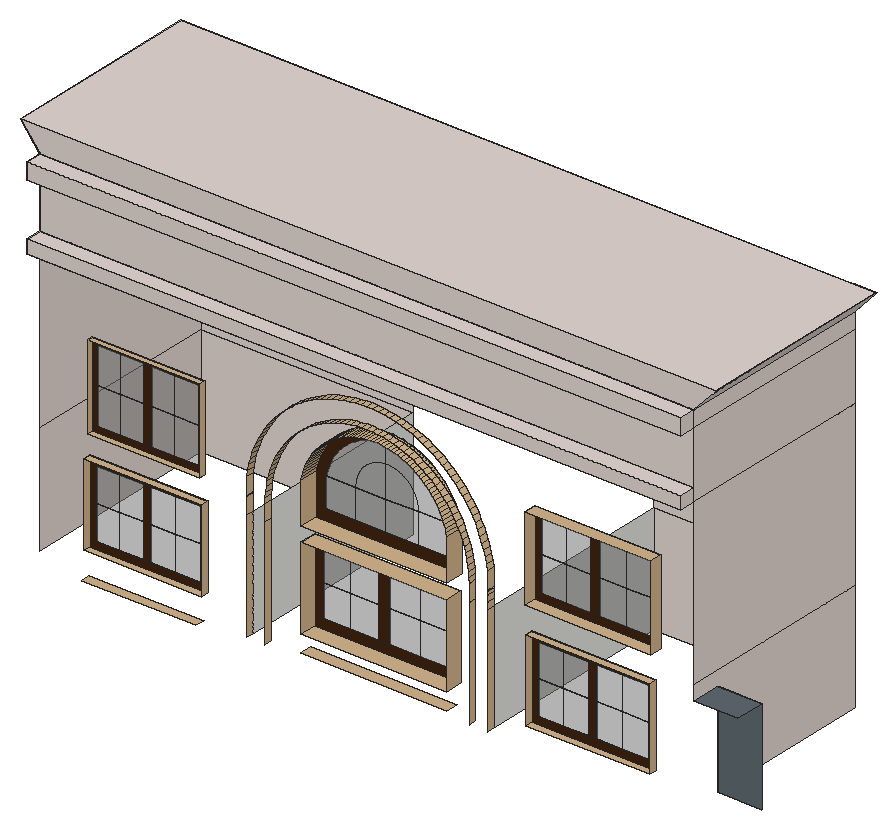
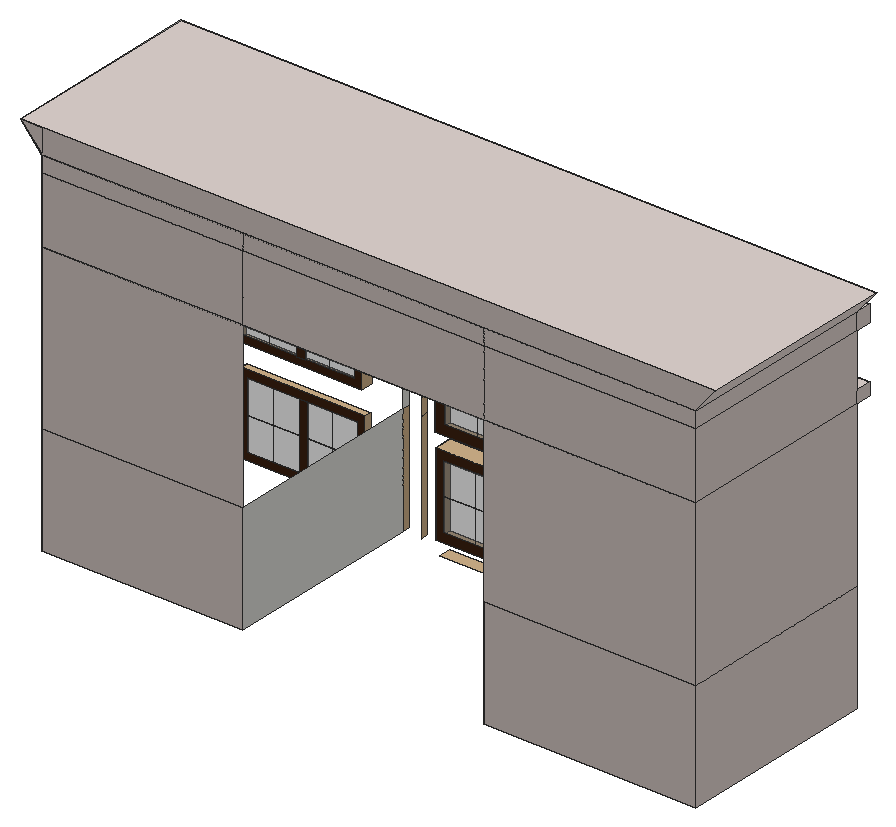
# SketchUp Ruby script. Lengths in inches.
U = 1.inch
M = Sketchup.active_model
def pt(a) = Geom::Point3d.new(a.map { |v| v * U })
def face(e, loops, mat)
  f = e.add_face(loops[0].map { |a| pt(a) })
  loops[1..].each { |l| e.add_face(l.map { |a| pt(a) }).erase! }
  f.material = f.back_material = mat if mat
  f
end
# faces: each face lists its corners as indices into pts; further lists are holes
def faces(e, pts, list, mat = nil) = list.each { |f| face(e, (f[0].is_a?(Array) ? f : [f]).map { |l| l.map { |i| pts[i] } }, mat) }
# xy, xz, yz: faces in a plane at the given z, y or x. An outline is a flat list of corners, or four numbers for a rectangle; further outlines are holes
def ring(l) = l.size == 4 ? [[l[0], l[1]], [l[2], l[1]], [l[2], l[3]], [l[0], l[3]]] : l.each_slice(2).to_a
def flat(e, list, mat, &to3) = list.each { |f| face(e, (f[0].is_a?(Array) ? f : [f]).map { |l| ring(l).map { |u, v| to3.(u, v) } }, mat) }
def xy(e, z, list, mat = nil) = flat(e, list, mat) { |x, y| [x, y, z] }
def xz(e, y, list, mat = nil) = flat(e, list, mat) { |x, z| [x, y, z] }
def yz(e, x, list, mat = nil) = flat(e, list, mat) { |y, z| [x, y, z] }
def lines(e, pts, list) = list.each { |a, b| e.add_line(pt(pts[a]), pt(pts[b])) }
# prism: a flat outline (further loops are holes) pulled along v
def prism(e, loops, v, mat = nil)
  f = face(e, loops, mat); d = Geom::Vector3d.new(v.map { |x| x * U })
  f.pushpull(f.normal.samedirection?(d) ? d.length : -d.length)
end
def box(e, o, s, mat = nil) = prism(e, [[o, [o[0] + s[0], o[1], o[2]], [o[0] + s[0], o[1] + s[1], o[2]], [o[0], o[1] + s[1], o[2]]]], [0, 0, s[2]], mat)
def at(x, y, z, deg = 0) = Geom::Transformation.translation(pt([x, y, z])) * Geom::Transformation.rotation(ORIGIN, Z_AXIS, deg.degrees)
def axes(o, x, y, z) = Geom::Transformation.new([*x, 0, *y, 0, *z, 0, *pt(o).to_a, 1])
def part(name) = M.definitions.add(name)
# library, detail: a bought-in or finely detailed component or shape, given as its bounding box
def library(name, o, s) = part(name).tap { |d| box(d.entities, o, s) }
def detail(e, o, s) = box(e.add_group.entities, o, s)
def put(e, d, t, mat = nil) = e.add_instance(d, t).tap { |i| i.material = mat if mat }
def group(e, t, mat = nil) = e.add_group.tap { |g| g.transformation = t; g.material = mat if mat }.entities
root = M.entities
M.materials.add("[0035_Tan]").color = [210, 180, 140]
M.materials.add("[Concrete Block 8x8 Gray]").color = [226, 214, 209]
M.materials.add("[Formica Speckled Grey]").color = [94, 105, 111]
M.materials.add("[Translucent Glass Gray]").color = [128, 128, 128]
M.materials["[Translucent Glass Gray]"].alpha = 0.5
M.materials.add("[Wood Cherry Original]").color = [66, 37, 18]
M.materials.add("[Wood Cherry Original]1").color = [66, 37, 18]
xy(root,250.26,[[47.15,148.73,134.71,155.98]],"[0035_Tan]")
xy(root,259.4,[[215.4,148.73,327.53,158.04]],"[0035_Tan]")
xy(root,270.29,[[387.81,148.73,483.43,154.29]],"[0035_Tan]")
xy(root,271.61,[[48.61,148.73,139.11,154.35]],"[0035_Tan]")
xy(root,272.4,[[215.4,148.73,327.53,162.23]],"[0035_Tan]")
xy(root,332.73,[[387.81,148.73,483.43,154.29]],"[0035_Tan]")
xy(root,332.73,[[516.88,148.73,550.94,171.42]],"[Formica Speckled Grey]")
xy(root,334.67,[[48.61,148.73,139.11,154.35]],"[0035_Tan]")
xy(root,335.78,[[215.4,148.73,327.53,162.23]],"[0035_Tan]")
xy(root,346.9,[[215.4,148.73,327.53,163.17]],"[0035_Tan]")
xy(root,352.68,[[387.3,148.73,484.24,158.23]],"[0035_Tan]")
xy(root,352.89,[[51.46,148.73,137.53,153.48]],"[0035_Tan]")
xy(root,417.08,[[51.46,148.73,137.53,153.48]],"[0035_Tan]")
xy(root,417.24,[[387.3,148.73,484.24,158.23]],"[0035_Tan]")
xy(root,469.3125,[[15.125,148.73,516.88,302.95]])
xy(root,469.3125,[[15.125,136.17,516.88,148.73]],"[Concrete Block 8x8 Gray]")
xy(root,479.24,[[15.125,136.17,516.88,148.73]],"[Concrete Block 8x8 Gray]")
xy(root,519.9375,[[15.125,136.17,516.88,148.73],[15.125,148.73,516.88,302.95]])
xy(root,532.5625,[[15.125,148.73,516.88,302.95]])
xy(root,532.5625,[[15.125,136.17,516.88,148.73]],"[Concrete Block 8x8 Gray]")
xy(root,551.1875,[[533.63,148.73,533.65,302.95]])
xy(root,551.375,[[0,148.73,533.63,302.95]],"[Concrete Block 8x8 Gray]")
xz(root,136.17,[[15.125,469.3125,516.88,479.24],[15.125,519.9375,516.88,532.5625]],"[Concrete Block 8x8 Gray]")
xz(root,148.73,[[178.17,343.6875,178.15,356.6,177.97,353.85,177.93,348.77],[178.17,343.6875,178.17,356.93,178.15,356.6],[363.16,343.6875,363.18,356.6,363.16,356.93],[363.16,343.6875,363.39,348.77,363.35,353.85,363.18,356.6],[178.15,356.6,178.17,356.93,178.17,370.47,178.125,370.32],
  [363.18,356.6,363.2,370.32,363.16,370.47,363.16,356.93],[15.125,469.3125,516.88,479.24],[15.125,519.9375,516.88,532.5625]])
xz(root,148.73,[[15.125,479.24,516.88,519.9375],[15.125,532.5625,516.88,532.5625,533.65,551.1875,533.63,551.1875,533.63,551.375,0,551.375]],"[Concrete Block 8x8 Gray]")
xz(root,153.48,[[55.61,357.04,73.22,384.98],[73.22,357.04,90.83,384.98],[96.95,357.04,115.16,384.98],[115.16,357.04,133.38,384.98],[55.61,384.98,73.22,412.93],
  [73.22,384.98,90.83,412.93],[96.95,384.98,115.16,412.93],[115.16,384.98,133.38,412.93]],"[Translucent Glass Gray]")
xz(root,153.48,[[[51.46,352.89,137.53,417.08],[55.61,357.04,133.38,412.93]],[90.83,357.04,96.95,412.93]],"[Wood Cherry Original]")
xz(root,154.29,[[393.42,275.91,412.77,301.51],[412.77,275.91,432.12,301.51],[437.78,275.91,457.8,301.51],[457.8,275.91,477.82,301.51],[393.42,301.51,412.77,327.12],
  [412.77,301.51,432.12,327.12],[437.78,301.51,457.8,327.12],[457.8,301.51,477.82,327.12]],"[Translucent Glass Gray]")
xz(root,154.29,[[[387.81,270.29,483.43,332.73],[393.42,275.91,477.82,327.12]],[432.12,275.91,437.78,327.12]],"[Wood Cherry Original]")
xz(root,154.35,[[53.95,276.94,72.21,303.14],[72.21,276.94,90.47,303.14],[95.58,276.94,114.68,303.14],[114.68,276.94,133.78,303.14],[53.95,303.14,72.21,329.33],
  [72.21,303.14,90.47,329.33],[95.58,303.14,114.68,329.33],[114.68,303.14,133.78,329.33]],"[Translucent Glass Gray]")
xz(root,154.35,[[[48.61,271.61,139.11,334.67],[53.95,276.94,133.78,329.33]],[90.47,276.94,95.58,329.33]],"[Wood Cherry Original]")
xz(root,158.23,[[392.69,358.07,411.63,384.96],[411.63,358.07,430.57,384.96],[437.11,358.07,457.98,384.96],[457.98,358.07,478.85,384.96],[392.69,384.96,411.63,411.85],
  [411.63,384.96,430.57,411.85],[437.11,384.96,457.98,411.85],[457.98,384.96,478.85,411.85]],"[Translucent Glass Gray]")
xz(root,158.23,[[[387.3,352.68,484.24,417.24],[392.69,358.07,478.85,411.85]],[430.57,358.07,437.11,411.85]],"[Wood Cherry Original]")
xz(root,162.23,[[222.14,279.14,243.24,304.09],[243.24,279.14,264.34,304.09],[272.89,279.14,296.84,304.09],[296.84,279.14,320.79,304.09],[222.14,304.09,243.24,329.04],
  [243.24,304.09,264.34,329.04],[272.89,304.09,296.84,329.04],[296.84,304.09,320.79,329.04]],"[Translucent Glass Gray]")
xz(root,162.23,[[[215.4,272.4,327.53,335.78],[222.14,279.14,320.79,329.04]]],"[Wood Cherry Original]")
xz(root,162.23,[[264.34,279.14,272.89,329.04]],"[Wood Cherry Original]1")
xz(root,163.17,[[223.26,354.76,246.24,377.71],[246.24,354.76,269.21,377.71],[269.21,354.76,294.44,377.71],[294.44,354.76,319.67,377.71],[223.26,377.71,246.24,377.71,246.24,378.32,246.27,378.93,246.31,379.54,246.36,380.15,246.43,380.76,246.52,381.37,246.62,381.97,246.73,382.57,246.86,383.17,247.01,383.76,247.17,384.35,247.35,384.9375,247.54,385.52,247.74,386.1,247.96,386.67,248.2,387.23,248.45,387.79,248.71,388.35,248.99,388.89,249.28,389.43,249.58,389.96,249.9,390.48,250.23,391,250.93,392,251.3,392.49,251.68,392.97,252.08,393.4375,252.48,393.9,252.9,394.34,253.33,394.78,253.77,395.21,254.22,395.625,254.68,396.03,255.15,396.42,255.63,396.8,256.12,397.17,256.62,397.52,257.125,397.86,257.64,398.19,258.16,398.51,258.7,398.8125,259.24,399.1,259.78,399.375,260.34,399.64,261.46,400.12,262.03,400.33,262.61,400.54,263.19,400.73,263.78,400.9,264.37,401.06,264.97,401.2,265.57,401.33,266.17,401.45,266.77,401.54,267.38,401.625,267.99,401.69,268.6,401.75,269.21,401.66,269.21,416.48,266.96,416.33,264.73,416.07,262.5,415.71,260.29,415.25,258.11,414.69,255.96,414.03,253.83,413.27,251.75,412.42,249.7,411.47,247.7,410.43,245.75,409.3,243.86,408.09,242.02,406.78,240.24,405.4,238.53,403.93,236.89,402.39,235.3125,400.78,233.82,399.09,232.4,397.34,231.06,395.52,229.8125,393.65,228.65,391.72,227.57,389.74,226.59,387.71,225.7,385.64,224.9,383.53,224.2,381.39,223.6,379.22],
  [246.24,377.71,269.21,377.71,269.21,401.66,268.6,401.75,267.99,401.69,267.38,401.625,266.77,401.54,266.17,401.45,265.57,401.33,264.97,401.2,264.37,401.06,263.78,400.9,263.19,400.73,262.61,400.54,262.03,400.33,261.46,400.12,260.34,399.64,259.78,399.375,259.24,399.1,258.7,398.8125,258.16,398.51,257.64,398.19,257.125,397.86,256.62,397.52,256.12,397.17,255.63,396.8,255.15,396.42,254.68,396.03,254.22,395.625,253.77,395.21,253.33,394.78,252.9,394.34,252.48,393.9,252.08,393.4375,251.68,392.97,251.3,392.49,250.93,392,250.23,391,249.9,390.48,249.58,389.96,249.28,389.43,248.99,388.89,248.71,388.35,248.45,387.79,248.2,387.23,247.96,386.67,247.74,386.1,247.54,385.52,247.35,384.9375,247.17,384.35,247.01,383.76,246.86,383.17,246.73,382.57,246.62,381.97,246.52,381.37,246.43,380.76,246.36,380.15,246.31,379.54,246.27,378.93,246.24,378.32],[269.21,377.71,294.44,377.71,294.43,378.36,294.41,379.01,294.36,379.65,294.3,380.3,294.22,380.95,294.13,381.59,294.01,382.23,293.88,382.87,293.74,383.5,293.57,384.125,293.39,384.75,293.19,385.37,292.98,385.98,292.75,386.59,292.5,387.19,292.23,387.79,291.95,388.37,291.66,388.95,291.35,389.52,291.02,390.08,290.68,390.64,290.32,391.18,289.95,391.71,289.57,392.24,289.17,392.75,288.76,393.25,288.33,393.74,287.89,394.22,287.44,394.69,286.98,395.15,286.5,395.59,286.01,396.02,285.51,396.43,285,396.84,284.48,397.22,283.95,397.6,283.41,397.96,282.86,398.3,282.3,398.63,281.73,398.95,281.15,399.25,280.57,399.53,279.98,399.8,279.38,400.05,278.77,400.29,278.16,400.5,277.54,400.71,276.92,400.89,276.29,401.0625,275.66,401.21,275.03,401.35,274.39,401.47,273.74,401.57,273.1,401.65,272.45,401.72,271.81,401.76,271.16,401.8,270.51,401.81,269.86,401.8,269.21,401.66],[294.44,377.71,319.67,377.71,319.33,379.22,318.73,381.39,318.03,383.53,317.23,385.64,316.34,387.71,315.36,389.74,314.28,391.72,313.12,393.65,311.87,395.52,310.53,397.34,309.11,399.09,307.62,400.78,306.05,402.39,304.4,403.93,302.69,405.4,300.91,406.78,299.07,408.09,297.18,409.3,295.23,410.43,293.23,411.47,291.18,412.42,289.1,413.27,286.98,414.03,284.82,414.69,282.64,415.25,280.43,415.71,278.21,416.07,275.97,416.33,273.72,416.48,271.47,416.53,269.21,416.48,269.21,401.66,269.86,401.8,270.51,401.81,271.16,401.8,271.81,401.76,272.45,401.72,273.1,401.65,273.74,401.57,274.39,401.47,275.03,401.35,275.66,401.21,276.29,401.0625,276.92,400.89,277.54,400.71,278.16,400.5,278.77,400.29,279.38,400.05,279.98,399.8,280.57,399.53,281.15,399.25,281.73,398.95,282.3,398.63,282.86,398.3,283.41,397.96,283.95,397.6,284.48,397.22,285,396.84,285.51,396.43,286.01,396.02,286.5,395.59,286.98,395.15,287.44,394.69,287.89,394.22,288.33,393.74,288.76,393.25,289.17,392.75,289.57,392.24,289.95,391.71,290.32,391.18,290.68,390.64,291.02,390.08,291.35,389.52,291.66,388.95,291.95,388.37,292.23,387.79,292.5,387.19,292.75,386.59,292.98,385.98,293.19,385.37,293.39,384.75,293.57,384.125,293.74,383.5,293.88,382.87,294.01,382.23,294.13,381.59,294.22,380.95,294.3,380.3,294.36,379.65,294.41,379.01,294.43,378.36]],"[Translucent Glass Gray]")
xz(root,163.17,[[[215.4,346.9,327.53,346.9,327.53,378.59,326.95,381.14,326.25,383.65,325.44,386.14,324.52,388.58,323.49,390.98,322.35,393.33,321.1,395.63,319.75,397.86,318.3,400.04,316.75,402.14,315.11,404.17,313.375,406.125,311.55,408,309.65,409.79,307.66,411.48,305.6,413.09,303.47,414.6,301.27,416.01,299.01,417.32,296.69,418.53,294.32,419.625,291.91,420.61,289.44,421.49,286.95,422.26,284.42,422.91,281.86,423.4375,279.28,423.85,276.68,424.15,274.08,424.33,271.47,424.39,268.85,424.33,266.25,424.15,263.65,423.85,261.07,423.4375,258.52,422.91,255.99,422.26,253.49,421.49,251.03,420.61,248.61,419.625,246.24,418.53,243.92,417.32,241.66,416.01,239.46,414.6,237.33,413.09,235.27,411.48,233.28,409.79,231.38,408,229.56,406.125,227.82,404.17,226.18,402.14,224.63,400.04,223.18,397.86,221.83,395.63,220.58,393.33,219.44,390.98,218.41,388.58,217.49,386.14,216.68,383.65,215.98,381.14,215.4,378.59],[223.26,354.76,223.26,377.71,223.6,379.22,224.2,381.39,224.9,383.53,225.7,385.64,226.59,387.71,227.57,389.74,228.65,391.72,229.8125,393.65,231.06,395.52,232.4,397.34,233.82,399.09,235.3125,400.78,236.89,402.39,238.53,403.93,240.24,405.4,242.02,406.78,243.86,408.09,245.75,409.3,247.7,410.43,249.7,411.47,251.75,412.42,253.83,413.27,255.96,414.03,258.11,414.69,260.29,415.25,262.5,415.71,264.73,416.07,266.96,416.33,269.21,416.48,271.47,416.53,273.72,416.48,275.97,416.33,278.21,416.07,280.43,415.71,282.64,415.25,284.82,414.69,286.98,414.03,289.1,413.27,291.18,412.42,293.23,411.47,295.23,410.43,297.18,409.3,299.07,408.09,300.91,406.78,302.69,405.4,304.4,403.93,306.05,402.39,307.62,400.78,309.11,399.09,310.53,397.34,311.87,395.52,313.12,393.65,314.28,391.72,315.36,389.74,316.34,387.71,317.23,385.64,318.03,383.53,318.73,381.39,319.33,379.22,319.67,377.71,319.67,354.76]]],"[Wood Cherry Original]")
xz(root,171.42,[[516.88,259.6875,550.94,332.73]],"[Formica Speckled Grey]")
xz(root,302.95,[[15.125,259.6875,178.17,343.6875],[363.16,259.6875,516.88,343.6875],[15.125,343.6875,178.17,469.3125],[363.16,343.6875,516.88,469.3125],[15.125,469.3125,178.17,519.9375],
  [178.17,469.3125,363.16,519.9375],[363.16,469.3125,516.88,519.9375],[15.125,519.9375,178.17,532.5625],[178.17,519.9375,363.16,532.5625],[363.16,519.9375,516.88,532.5625],
  [15.125,532.5625,0,551.375,533.63,551.375,533.63,551.1875,516.88,551.1875,516.88,532.5625],[516.88,532.5625,516.88,551.1875,533.65,551.1875]],"[Concrete Block 8x8 Gray]")
yz(root,15.125,[[148.73,259.6875,302.95,343.6875],[148.73,343.6875,302.95,469.3125],[136.17,469.3125,148.73,479.24],[148.73,469.3125,302.95,519.9375],[136.17,519.9375,148.73,532.5625],
  [148.73,519.9375,302.95,532.5625]],"[Concrete Block 8x8 Gray]")
yz(root,48.61,[[148.73,271.61,154.35,334.67]],"[0035_Tan]")
yz(root,51.46,[[148.73,352.89,153.48,417.08]],"[0035_Tan]")
yz(root,137.53,[[148.73,352.89,153.48,417.08]],"[0035_Tan]")
yz(root,139.11,[[148.73,271.61,154.35,334.67]],"[0035_Tan]")
yz(root,178.17,[[148.73,259.6875,302.95,343.6875]])
yz(root,178.17,[[143.23,259.6875,148.73,343.6875],[143.23,343.6875,148.73,356.93],[143.23,356.93,148.73,370.47]],"[0035_Tan]")
yz(root,192.26,[[143.23,259.6875,148.73,343.6875],[143.23,343.6875,148.73,356.49]],"[0035_Tan]")
yz(root,215.4,[[148.73,272.4,162.23,335.78],[148.73,346.9,163.17,378.59]],"[0035_Tan]")
yz(root,327.53,[[148.73,272.4,162.23,335.78],[148.73,346.9,163.17,378.59]],"[0035_Tan]")
yz(root,349.07,[[143.23,259.6875,148.73,343.6875],[143.23,343.6875,148.73,356.49]],"[0035_Tan]")
yz(root,363.16,[[148.73,259.6875,302.95,343.6875],[143.23,343.6875,148.73,356.93]])
yz(root,363.16,[[143.23,259.6875,148.73,343.6875],[143.23,356.93,148.73,370.47]],"[0035_Tan]")
yz(root,387.3,[[148.73,352.68,158.23,417.24]],"[0035_Tan]")
yz(root,387.81,[[148.73,270.29,154.29,332.73]],"[0035_Tan]")
yz(root,483.43,[[148.73,270.29,154.29,332.73]],"[0035_Tan]")
yz(root,484.24,[[148.73,352.68,158.23,417.24]],"[0035_Tan]")
yz(root,516.88,[[171.42,259.6875,302.95,259.6875,302.95,343.6875,148.73,343.6875,148.73,332.73,171.42,332.73],[148.73,343.6875,302.95,469.3125],[136.17,469.3125,148.73,479.24],[148.73,469.3125,302.95,519.9375],[136.17,519.9375,148.73,532.5625],
  [148.73,519.9375,302.95,532.5625]],"[Concrete Block 8x8 Gray]")
yz(root,533.63,[[148.73,551.1875,302.95,551.375]])
p = [[178.17,148.73,343.6875],[177.93,148.73,348.77],[177.93,143.23,348.77],[178.17,143.23,343.6875],[178.15,148.73,356.6],[178.15,143.23,356.6],
  [363.16,148.73,343.6875],[363.18,148.73,356.6],[363.18,143.23,356.6],[363.16,143.23,343.6875],[363.39,148.73,348.77],[363.39,143.23,348.77],
  [177.97,148.73,353.85],[177.97,143.23,353.85],[363.35,148.73,353.85],[363.35,143.23,353.85],[192.26,148.73,356.49],[192.36,148.73,360.59],
  [192.36,143.23,360.59],[192.26,143.23,356.49],[348.96,148.73,360.59],[349.07,148.73,356.49],[349.07,143.23,356.49],[348.96,143.23,360.59],
  [192.6875,148.73,364.68],[192.6875,143.23,364.68],[348.64,148.73,364.68],[348.64,143.23,364.68],[193.22,148.73,368.75],[193.22,143.23,368.75],
  [348.1,148.73,368.75],[348.1,143.23,368.75],[193.97,148.73,372.79],[193.97,143.23,372.79],[347.36,148.73,372.79],[347.36,143.23,372.79],
  [178.88,148.73,374.86],[178.17,148.73,370.47],[178.17,143.23,370.47],[178.88,143.23,374.86],[363.16,148.73,370.47],[362.44,148.73,374.86],
  [362.44,143.23,374.86],[363.16,143.23,370.47],[194.93,148.73,376.78],[194.93,143.23,376.78],[346.4,148.73,376.78],[346.4,143.23,376.78],
  [179.83,148.73,379.2],[179.83,143.23,379.2],[361.49,148.73,379.2],[361.49,143.23,379.2],[196.09,148.73,380.72],[196.09,143.23,380.72],
  [345.23,148.73,380.72],[345.23,143.23,380.72],[215.98,148.73,381.14],[215.4,148.73,378.59],[215.4,163.17,378.59],[215.98,163.17,381.14],
  [327.53,148.73,378.59],[326.95,148.73,381.14],[326.95,163.17,381.14],[327.53,163.17,378.59],[180.98,148.73,383.5],[180.98,143.23,383.5],
  [360.34,148.73,383.5],[360.34,143.23,383.5],[197.46,148.73,384.59],[197.46,143.23,384.59],[343.86,148.73,384.59],[343.86,143.23,384.59],
  [216.68,148.73,383.65],[216.68,163.17,383.65],[326.25,148.73,383.65],[326.25,163.17,383.65],[182.34,148.73,387.74],[182.34,143.23,387.74],
  [358.99,148.73,387.74],[358.99,143.23,387.74],[217.49,148.73,386.14],[217.49,163.17,386.14],[325.44,148.73,386.14],[325.44,163.17,386.14],
  [199.03,148.73,388.38],[199.03,143.23,388.38],[342.29,148.73,388.38],[342.29,143.23,388.38],[218.41,148.73,388.58],[218.41,163.17,388.58],
  [324.52,148.73,388.58],[324.52,163.17,388.58],[183.89,148.73,391.91],[183.89,143.23,391.91],[357.43,148.73,391.91],[357.43,143.23,391.91],
  [200.8,148.73,392.08],[200.8,143.23,392.08],[340.52,148.73,392.08],[340.52,143.23,392.08],[219.44,148.73,390.98],[219.44,163.17,390.98],
  [323.49,148.73,390.98],[323.49,163.17,390.98],[220.58,148.73,393.33],[220.58,163.17,393.33],[322.35,148.73,393.33],[322.35,163.17,393.33],
  [185.64,148.73,395.99],[185.64,143.23,395.99],[355.68,148.73,395.99],[355.68,143.23,395.99],[202.76,148.73,395.69],[202.76,143.23,395.69],
  [338.56,148.73,395.69],[338.56,143.23,395.69],[221.83,148.73,395.63],[221.83,163.17,395.63],[321.1,148.73,395.63],[321.1,163.17,395.63],
  [223.18,148.73,397.86],[223.18,163.17,397.86],[319.75,148.73,397.86],[319.75,163.17,397.86],[204.91,148.73,399.19],[204.91,143.23,399.19],
  [336.42,148.73,399.19],[336.42,143.23,399.19],[187.59,148.73,400],[187.59,143.23,400],[353.74,148.73,400],[353.74,143.23,400],
  [224.63,148.73,400.04],[224.63,163.17,400.04],[318.3,148.73,400.04],[318.3,163.17,400.04],[207.23,148.73,402.57],[207.23,143.23,402.57],
  [334.1,148.73,402.57],[334.1,143.23,402.57],[189.72,148.73,403.9],[189.72,143.23,403.9],[351.6,148.73,403.9],[351.6,143.23,403.9],
  [226.18,148.73,402.14],[226.18,163.17,402.14],[316.75,148.73,402.14],[316.75,163.17,402.14],[227.82,148.73,404.17],[227.82,163.17,404.17],
  [315.11,148.73,404.17],[315.11,163.17,404.17],[209.73,148.73,405.83],[209.73,143.23,405.83],[331.6,148.73,405.83],[331.6,143.23,405.83],
  [192.04,148.73,407.7],[192.04,143.23,407.7],[349.29,148.73,407.7],[349.29,143.23,407.7],[229.56,148.73,406.125],[229.56,163.17,406.125],
  [313.375,148.73,406.125],[313.375,163.17,406.125],[212.4,148.73,408.95],[212.4,143.23,408.95],[328.93,148.73,408.95],[328.93,143.23,408.95],
  [231.38,148.73,408],[231.38,163.17,408],[311.55,148.73,408],[311.55,163.17,408],[194.53,148.73,411.38],[194.53,143.23,411.38],
  [346.8,148.73,411.38],[346.8,143.23,411.38],[233.28,148.73,409.79],[233.28,163.17,409.79],[309.65,148.73,409.79],[309.65,163.17,409.79],
  [215.22,148.73,411.93],[215.22,143.23,411.93],[326.1,148.73,411.93],[326.1,143.23,411.93],[235.27,148.73,411.48],[235.27,163.17,411.48],
  [307.66,148.73,411.48],[307.66,163.17,411.48],[197.2,148.73,414.94],[197.2,143.23,414.94],[344.13,148.73,414.94],[344.13,143.23,414.94],
  [237.33,148.73,413.09],[237.33,163.17,413.09],[305.6,148.73,413.09],[305.6,163.17,413.09],[218.2,148.73,414.76],[218.2,143.23,414.76],
  [323.13,148.73,414.76],[323.13,143.23,414.76],[239.46,148.73,414.6],[239.46,163.17,414.6],[303.47,148.73,414.6],[303.47,163.17,414.6],
  [241.66,148.73,416.01],[241.66,163.17,416.01],[301.27,148.73,416.01],[301.27,163.17,416.01],[221.32,148.73,417.42],[221.32,143.23,417.42],
  [320.01,148.73,417.42],[320.01,143.23,417.42],[200.03,148.73,418.37],[200.03,143.23,418.37],[341.3,148.73,418.37],[341.3,143.23,418.37],
  [243.92,148.73,417.32],[243.92,163.17,417.32],[299.01,148.73,417.32],[299.01,163.17,417.32],[246.24,148.73,418.53],[246.24,163.17,418.53],
  [296.69,148.73,418.53],[296.69,163.17,418.53],[224.58,148.73,419.92],[224.58,143.23,419.92],[316.75,148.73,419.92],[316.75,143.23,419.92],
  [203.02,148.73,421.66],[203.02,143.23,421.66],[338.3,148.73,421.66],[338.3,143.23,421.66],[248.61,148.73,419.625],[248.61,163.17,419.625],
  [294.32,148.73,419.625],[294.32,163.17,419.625],[251.03,148.73,420.61],[251.03,163.17,420.61],[291.91,148.73,420.61],[291.91,163.17,420.61],
  [227.96,148.73,422.25],[227.96,143.23,422.25],[313.37,148.73,422.25],[313.37,143.23,422.25],[253.49,148.73,421.49],[253.49,163.17,421.49],
  [289.44,148.73,421.49],[289.44,163.17,421.49],[255.99,148.73,422.26],[255.99,163.17,422.26],[286.95,148.73,422.26],[286.95,163.17,422.26],
  [206.17,148.73,424.81],[206.17,143.23,424.81],[335.16,148.73,424.81],[335.16,143.23,424.81],[231.46,148.73,424.39],[231.46,143.23,424.39],
  [309.87,148.73,424.39],[309.87,143.23,424.39],[258.52,148.73,422.91],[258.52,163.17,422.91],[284.42,148.73,422.91],[284.42,163.17,422.91],
  [261.07,148.73,423.4375],[261.07,163.17,423.4375],[281.86,148.73,423.4375],[281.86,163.17,423.4375],[263.65,148.73,423.85],[263.65,163.17,423.85],
  [279.28,148.73,423.85],[279.28,163.17,423.85],[266.25,148.73,424.15],[266.25,163.17,424.15],[276.68,148.73,424.15],[276.68,163.17,424.15],
  [268.85,148.73,424.33],[268.85,163.17,424.33],[274.08,148.73,424.33],[274.08,163.17,424.33],[271.47,148.73,424.39],[271.47,163.17,424.39],
  [235.07,148.73,426.35],[235.07,143.23,426.35],[306.26,148.73,426.35],[306.26,143.23,426.35],[209.46,148.73,427.8],[209.46,143.23,427.8],
  [331.87,148.73,427.8],[331.87,143.23,427.8],[238.77,148.73,428.12],[238.77,143.23,428.12],[302.55,148.73,428.12],[302.55,143.23,428.12],
  [212.89,148.73,430.63],[212.89,143.23,430.63],[328.4375,148.73,430.63],[328.4375,143.23,430.63],[242.5625,148.73,429.6875],[242.5625,143.23,429.6875],
  [298.76,148.73,429.6875],[298.76,143.23,429.6875],[246.43,148.73,431.06],[246.43,143.23,431.06],[294.89,148.73,431.06],[294.89,143.23,431.06],
  [216.45,148.73,433.3],[216.45,143.23,433.3],[324.875,148.73,433.3],[324.875,143.23,433.3],[250.37,148.73,432.22],[250.37,143.23,432.22],
  [290.96,148.73,432.22],[290.96,143.23,432.22],[254.36,148.73,433.18],[254.36,143.23,433.18],[286.96,148.73,433.18],[286.96,143.23,433.18],
  [258.4,148.73,433.93],[258.4,143.23,433.93],[282.93,148.73,433.93],[282.93,143.23,433.93],[220.13,148.73,435.79],[220.13,143.23,435.79],
  [321.19,148.73,435.79],[321.19,143.23,435.79],[262.47,148.73,434.47],[262.47,143.23,434.47],[278.86,148.73,434.47],[278.86,143.23,434.47],
  [266.56,148.73,434.79],[266.56,143.23,434.79],[274.77,148.73,434.79],[274.77,143.23,434.79],[270.66,148.73,434.89],[270.66,143.23,434.89],
  [223.93,148.73,438.11],[223.93,143.23,438.11],[317.39,148.73,438.11],[317.39,143.23,438.11],[227.84,148.73,440.24],[227.84,143.23,440.24],
  [313.49,148.73,440.24],[313.49,143.23,440.24],[231.84,148.73,442.18],[231.84,143.23,442.18],[309.49,148.73,442.18],[309.49,143.23,442.18],
  [235.93,148.73,443.93],[235.93,143.23,443.93],[305.4,148.73,443.93],[305.4,143.23,443.93],[240.09,148.73,445.49],[240.09,143.23,445.49],
  [301.23,148.73,445.49],[301.23,143.23,445.49],[244.33,148.73,446.84],[244.33,143.23,446.84],[296.99,148.73,446.84],[296.99,143.23,446.84],
  [248.63,148.73,447.99],[248.63,143.23,447.99],[292.7,148.73,447.99],[292.7,143.23,447.99],[252.98,148.73,448.9375],[252.98,143.23,448.9375],
  [288.35,148.73,448.9375],[288.35,143.23,448.9375],[257.36,148.73,449.67],[257.36,143.23,449.67],[283.96,148.73,449.67],[283.96,143.23,449.67],
  [261.78,148.73,450.2],[261.78,143.23,450.2],[279.55,148.73,450.2],[279.55,143.23,450.2],[266.22,148.73,450.52],[266.22,143.23,450.52],
  [275.11,148.73,450.52],[275.11,143.23,450.52],[270.66,148.73,450.625],[270.66,143.23,450.625],[15.125,148.73,532.5625],[0,148.73,551.375],
  [0,302.95,551.375],[15.125,302.95,532.5625],[533.65,148.73,551.1875],[516.88,148.73,532.5625],[516.88,302.95,532.5625],[533.65,302.95,551.1875]]
faces(root,p,[[0,1,2,3],[10,6,9,11],[1,12,13,2],[14,10,11,15],[12,4,5,13],[7,14,15,8],[16,17,18,19],[20,21,22,23],
  [17,24,25,18],[26,20,23,27],[24,28,29,25],[30,26,27,31],[28,32,33,29],[34,30,31,35],[36,37,38,39],[40,41,42,43],
  [32,44,45,33],[46,34,35,47],[48,36,39,49],[41,50,51,42],[44,52,53,45],[54,46,47,55],[56,57,58,59],[60,61,62,63],
  [64,48,49,65],[50,66,67,51],[52,68,69,53],[70,54,55,71],[72,56,59,73],[61,74,75,62],[76,64,65,77],[66,78,79,67],
  [80,72,73,81],[74,82,83,75],[68,84,85,69],[86,70,71,87],[88,80,81,89],[82,90,91,83],[92,76,77,93],[78,94,95,79],
  [84,96,97,85],[98,86,87,99],[100,88,89,101],[90,102,103,91],[104,100,101,105],[102,106,107,103],[108,92,93,109],[94,110,111,95],
  [96,112,113,97],[114,98,99,115],[116,104,105,117],[106,118,119,107],[120,116,117,121],[118,122,123,119],[112,124,125,113],[126,114,115,127],
  [128,108,109,129],[110,130,131,111],[132,120,121,133],[122,134,135,123],[124,136,137,125],[138,126,127,139],[140,128,129,141],[130,142,143,131],
  [144,132,133,145],[134,146,147,135],[148,144,145,149],[146,150,151,147],[136,152,153,137],[154,138,139,155],[156,140,141,157],[142,158,159,143],
  [160,148,149,161],[150,162,163,151],[152,164,165,153],[166,154,155,167],[168,160,161,169],[162,170,171,163],[172,156,157,173],[158,174,175,159],
  [176,168,169,177],[170,178,179,171],[164,180,181,165],[182,166,167,183],[184,176,177,185],[178,186,187,179],[188,172,173,189],[174,190,191,175],
  [192,184,185,193],[186,194,195,187],[180,196,197,181],[198,182,183,199],[200,192,193,201],[194,202,203,195],[204,200,201,205],[202,206,207,203],
  [196,208,209,197],[210,198,199,211],[212,188,189,213],[190,214,215,191],[216,204,205,217],[206,218,219,207],[220,216,217,221],[218,222,223,219],
  [208,224,225,209],[226,210,211,227],[228,212,213,229],[214,230,231,215],[232,220,221,233],[222,234,235,223],[236,232,233,237],[234,238,239,235],
  [224,240,241,225],[242,226,227,243],[244,236,237,245],[238,246,247,239],[248,244,245,249],[246,250,251,247],[252,228,229,253],[230,254,255,231],
  [240,256,257,241],[258,242,243,259],[260,248,249,261],[250,262,263,251],[264,260,261,265],[262,266,267,263],[268,264,265,269],[266,270,271,267],
  [272,268,269,273],[270,274,275,271],[276,272,273,277],[274,278,279,275],[280,276,277,281],[278,280,281,279],[256,282,283,257],[284,258,259,285],
  [286,252,253,287],[254,288,289,255],[282,290,291,283],[292,284,285,293],[294,286,287,295],[288,296,297,289],[290,298,299,291],[300,292,293,301],
  [298,302,303,299],[304,300,301,305],[306,294,295,307],[296,308,309,297],[302,310,311,303],[312,304,305,313],[310,314,315,311],[316,312,313,317],
  [314,318,319,315],[320,316,317,321],[322,306,307,323],[308,324,325,309],[318,326,327,319],[328,320,321,329],[326,330,331,327],[332,328,329,333],
  [330,334,335,331],[334,332,333,335],[336,322,323,337],[324,338,339,325],[340,336,337,341],[338,342,343,339],[344,340,341,345],[342,346,347,343],
  [348,344,345,349],[346,350,351,347],[352,348,349,353],[350,354,355,351],[356,352,353,357],[354,358,359,355],[360,356,357,361],[358,362,363,359],
  [364,360,361,365],[362,366,367,363],[368,364,365,369],[366,370,371,367],[372,368,369,373],[370,374,375,371],[376,372,373,377],[374,378,379,375],
  [380,376,377,381],[378,380,381,379]],"[0035_Tan]")
faces(root,p,[[4,0,3,5],[6,7,8,9]])
faces(root,p,[[382,383,384,385],[386,387,388,389]],"[Concrete Block 8x8 Gray]")
